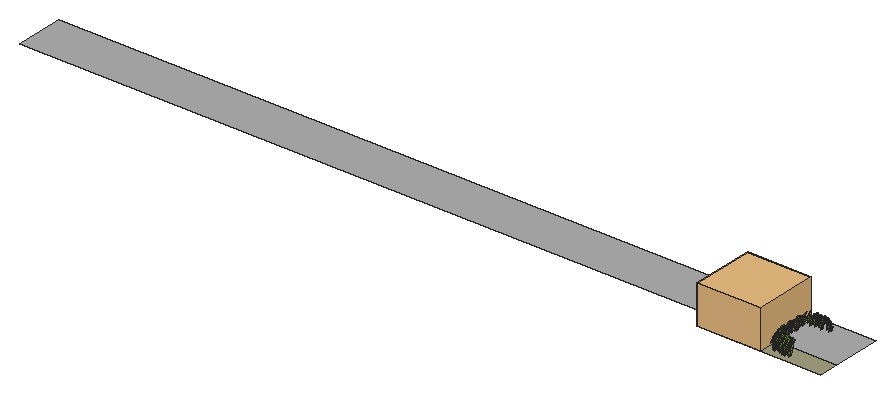
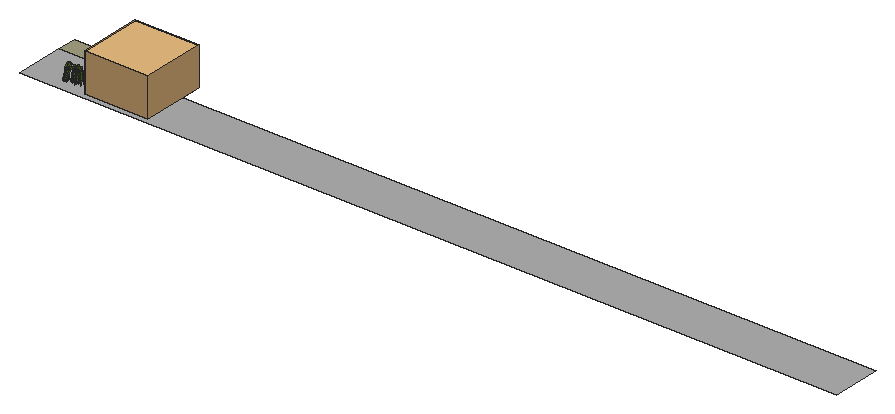
# SketchUp Ruby script. Lengths in inches.
U = 1.inch
M = Sketchup.active_model
def pt(a) = Geom::Point3d.new(a.map { |v| v * U })
def face(e, loops, mat)
  f = e.add_face(loops[0].map { |a| pt(a) })
  loops[1..].each { |l| e.add_face(l.map { |a| pt(a) }).erase! }
  f.material = f.back_material = mat if mat
  f
end
# faces: each face lists its corners as indices into pts; further lists are holes
def faces(e, pts, list, mat = nil) = list.each { |f| face(e, (f[0].is_a?(Array) ? f : [f]).map { |l| l.map { |i| pts[i] } }, mat) }
# xy, xz, yz: faces in a plane at the given z, y or x. An outline is a flat list of corners, or four numbers for a rectangle; further outlines are holes
def ring(l) = l.size == 4 ? [[l[0], l[1]], [l[2], l[1]], [l[2], l[3]], [l[0], l[3]]] : l.each_slice(2).to_a
def flat(e, list, mat, &to3) = list.each { |f| face(e, (f[0].is_a?(Array) ? f : [f]).map { |l| ring(l).map { |u, v| to3.(u, v) } }, mat) }
def xy(e, z, list, mat = nil) = flat(e, list, mat) { |x, y| [x, y, z] }
def xz(e, y, list, mat = nil) = flat(e, list, mat) { |x, z| [x, y, z] }
def yz(e, x, list, mat = nil) = flat(e, list, mat) { |y, z| [x, y, z] }
def lines(e, pts, list) = list.each { |a, b| e.add_line(pt(pts[a]), pt(pts[b])) }
# prism: a flat outline (further loops are holes) pulled along v
def prism(e, loops, v, mat = nil)
  f = face(e, loops, mat); d = Geom::Vector3d.new(v.map { |x| x * U })
  f.pushpull(f.normal.samedirection?(d) ? d.length : -d.length)
end
def box(e, o, s, mat = nil) = prism(e, [[o, [o[0] + s[0], o[1], o[2]], [o[0] + s[0], o[1] + s[1], o[2]], [o[0], o[1] + s[1], o[2]]]], [0, 0, s[2]], mat)
def at(x, y, z, deg = 0) = Geom::Transformation.translation(pt([x, y, z])) * Geom::Transformation.rotation(ORIGIN, Z_AXIS, deg.degrees)
def axes(o, x, y, z) = Geom::Transformation.new([*x, 0, *y, 0, *z, 0, *pt(o).to_a, 1])
def part(name) = M.definitions.add(name)
# library, detail: a bought-in or finely detailed component or shape, given as its bounding box
def library(name, o, s) = part(name).tap { |d| box(d.entities, o, s) }
def detail(e, o, s) = box(e.add_group.entities, o, s)
def put(e, d, t, mat = nil) = e.add_instance(d, t).tap { |i| i.material = mat if mat }
def group(e, t, mat = nil) = e.add_group.tap { |g| g.transformation = t; g.material = mat if mat }.entities
root = M.entities
M.materials.add("[0061_OliveDrab]").color = [107, 142, 35]
M.materials.add("[Carrera Marble]").color = [175, 175, 175]
M.materials.add("[Stone Coursed Rough]").color = [165, 160, 130]
c1 = library("Ornamental grass",[0,0,0],[38.24,37.94,23.16])
xy(root,543.57,[[507.27,12.12,581.95,12.12,582,41.21,90,42,89.95,12.79]],"[Carrera Marble]")
xy(root,543.57,[[581.93,0,581.95,12,581.95,12.12,507.27,12.12,507.25,0.12]],"[Stone Coursed Rough]")
p = [[554.875,33.375,546.1875],[555.06,33.4,546.1875],[554.94,33.55,543.57],[559.39,33.72,546.375],[559.6,33.65,546.375],[559.56,33.87,543.76],
  [548.13,13.96,546.65],[548.03,14.16,546.65],[547.88,13.96,544.03],[554.52,3.95,546.7],[554.3,3.97,546.7],[554.38,3.71,544.08],
  [552.98,4.9,546.76],[552.83,5.02,546.76],[552.8125,4.84,544.14],[547.99,17.08,546.71],[548,17.28,546.71],[547.83,17.1875,544.09],
  [547.81,25.01,546.74],[547.76,25.22,546.74],[547.56,25.05,544.125],[551.43,33.03,546.84],[551.61,33.14,546.84],[551.34,33.36,544.23],
  [558.59,34.56,546.78],[558.8125,34.54,546.78],[558.74,34.99,544.19],[547.64,10.6875,546.94],[547.66,10.89,546.94],[547.33,10.82,544.34],
  [555.98,33.58,546.87],[556.18,33.64,546.87],[556.02,33.8,544.26],[559.47,34.28,546.91],[559.65,34.36,546.91],[559.375,34.74,544.33],
  [560.17,34.34,546.875],[560.34,34.28,546.875],[560.42,34.74,544.29],[558.55,2.88,546.9375],[558.37,2.88,546.9375],[558.46,2.25,544.39],
  [548.33,7,546.97],[548.21,7.16,546.97],[547.78,6.72,544.42],[547.35,24.36,546.96],[547.3125,24.5625,546.96],[547.01,24.4,544.35],
  [549.7,32.17,547.01],[549.83,32.29,547.01],[549.45,32.56,544.43],[556.84,3.7,547.19],[556.625,3.77,547.19],[556.625,3.39,544.59],
  [547.6875,12.91,547.21],[547.71,13.11,547.21],[547.47,13.04,544.6],[553.87,33.84,547.23],[554.09,33.87,547.23],[553.94,34.17,544.62],
  [547.98,25.15,547.28],[548.03,25.34,547.28],[547.84,25.28,544.66],[553.67,33.4375,547.29],[553.875,33.53,547.29],[553.67,33.71,544.68],
  [551.34,4.06,547.3],[551.18,4.2,547.3],[550.85,3.65,544.75],[547.21,12.875,547.33],[547.1,13.05,547.33],[546.66,12.67,544.77],
  [547.81,15.4,547.43],[547.82,15.6,547.43],[547.6,15.51,544.8125],[546.54,15.71,547.29],[546.59,15.89,547.29],[545.85,15.98,544.77],
  [547.69,19.24,547.4],[547.66,19.4375,547.4],[547.39,19.29,544.8],[546.58,22.72,547.41],[546.5625,22.91,547.41],[546.02,22.77,544.85],
  [549.64,31.94,547.39],[549.78,32.07,547.39],[549.41,32.33,544.8],[552.55,33.67,547.42],[552.73,33.81,547.42],[552.35,34.12,544.84],
  [557.29,2.375,547.39],[557.1,2.41,547.39],[557.03,1.54,544.91],[555.79,3.96,547.51],[555.58,4.04,547.51],[555.6,3.76,544.9],
  [546.99,11.17,547.49],[547.01,11.375,547.49],[546.49,11.33,544.92],[547.1,21.32,547.48],[547.125,21.51,547.48],[546.73,21.46,544.88],
  [547.73,29.28,547.47],[547.84,29.45,547.47],[547.41,29.61,544.88],[558.51,33.59,547.5625],[558.73,33.58,547.5625],[558.625,33.77,544.94],
  [558.98,3.64,547.66],[558.77,3.67,547.66],[558.84,3.38,545.05],[546.62,20.42,547.55],[546.58,20.64,547.55],[545.91,20.39,545.02],
  [550.37,32.24,547.62],[550.54,32.34,547.62],[550.3,32.5625,545.01],[552.85,34.23,547.56],[553.0625,34.28,547.56],[552.84,34.76,544.98],
  [558.88,34.69,547.61],[559.09,34.74,547.61],[558.87,35.16,545.03],[560.95,2.5625,547.61],[560.77,2.53,547.61],[560.97,1.85,545.08],
  [546.58,25.53,547.66],[546.6,25.74,547.66],[545.95,25.67,545.11],[555.14,4.24,547.79],[554.93,4.31,547.79],[554.98,4.1,545.17],
  [552.38,4.51,547.85],[552.1875,4.59,547.85],[552.1875,4.3125,545.24],[547.5625,11.58,547.79],[547.49,11.75,547.79],[547.16,11.51,545.2],
  [547.32,12.1875,547.78],[547.375,12.38,547.78],[546.92,12.42,545.2],[546.48,14.16,547.72],[546.48,14.36,547.72],[545.76,14.26,545.2],
  [547.77,20.79,547.79],[547.75,21.01,547.79],[547.51,20.89,545.18],[547.89,24.82,547.83],[547.82,25.02,547.83],[547.65,24.85,545.21],
  [552.85,33.28,547.77],[553.04,33.38,547.77],[552.84,33.53,545.16],[561,33.55,547.86],[561.21,33.5,547.86],[561.14,33.67,545.24],
  [558.03,2.67,547.8125],[557.8125,2.62,547.8125],[558.07,1.98,545.28],[552.3,4.71,547.87],[552.09,4.75,547.87],[552.15,4.46,545.26],
  [548.19,7.04,547.88],[548.07,7.21,547.88],[547.72,6.83,545.31],[547.51,25.92,547.94],[547.46,26.125,547.94],[547.16,25.93,545.34],
  [560.18,35.33,547.83],[560.38,35.32,547.83],[560.34,36.14,545.34],[557.6875,3.67,548.05],[557.49,3.71,548.05],[557.52,3.37,545.45],
  [548.57,8.09,548.03],[548.42,8.25,548.03],[548.26,7.95,545.42],[548.13,16.84,548.05],[548.1,17.07,548.05],[547.94,16.92,545.43],
  [546.64,28.21,547.88],[546.71,28.41,547.88],[545.96,28.57,545.375],[560.52,3.79,548.12],[560.32,3.78,548.12],[560.44,3.53,545.51],
  [556.02,3.8,548.11],[555.82,3.88,548.11],[555.8,3.55,545.51],[547.55,15.5,548.14],[547.53,15.6875,548.14],[547.26,15.5625,545.54],
  [546.82,22.12,548.03],[546.86,22.31,548.03],[546.36,22.32,545.45],[549.46,32.1,548.07],[549.6,32.21,548.07],[549.17,32.63,545.52],
  [561.73,3.14,548.15],[561.51,3.09,548.15],[561.73,2.64,545.58],[548.04,14,548.17],[547.96,14.18,548.17],[547.82,14.01,545.55],
  [547.98,27.52,548.17],[547.98,27.73,548.17],[547.75,27.63,545.56],[547.37,6.89,548.12],[547.27,7.0625,548.12],[546.45,6.45,545.7],
  [547.9,26.79,548.3],[548.01,26.95,548.3],[547.73,27.03,545.69],[559.3125,35.01,548.18],[559.52,34.95,548.18],[559.59,35.68,545.66],
  [546.42,9.09,548.23],[546.38,9.3,548.23],[545.5625,9.03,545.75],[546.4,23.11,548.3],[546.4,23.33,548.3],[545.73,23.2,545.76],
  [547.9375,32.03,548.18],[548.04,32.21,548.18],[547.05,32.65,545.79],[552.25,33.93,548.41],[552.4375,33.98,548.41],[552.2,34.47,545.84],
  [558.33,35.84,548.2],[558.53,35.89,548.2],[558.21,36.91,545.81],[553.34,2.23,548.25],[553.14,2.26,548.25],[553.09,1.16,545.86],
  [560.92,2.53,548.47],[560.71,2.56,548.47],[560.73,1.89,545.93],[558.86,3.11,548.46],[558.67,3.16,548.46],[558.63,2.68,545.88],
  [557.57,2.04,548.47],[557.37,2.02,548.47],[557.54,1.23,545.98],[551.75,3.56,548.45],[551.54,3.62,548.45],[551.41,2.78,545.96],
  [557.97,3.76,548.6],[557.77,3.8,548.6],[557.83,3.52,545.98],[560.29,3.72,548.61],[560.1,3.73,548.61],[560.1875,3.48,546],
  [548.51,7.28,548.57],[548.39,7.47,548.57],[548.07,7.125,545.98],[548.29,14.96,548.61],[548.2,15.125,548.61],[548.11,14.96,545.99],
  [546.84,26.42,548.56],[546.86,26.64,548.56],[546.39,26.58,545.97],[555.38,35.11,548.5625],[555.58,35.1875,548.5625],[555.21,35.84,546.05],
  [552.23,2.64,548.52],[552.0625,2.76,548.52],[551.5,1.79,546.15],[546.44,20.76,548.62],[546.41,20.96,548.62],[545.69,20.75,546.1],
  [546.01,24.9,548.47],[546.08,25.08,548.47],[545.06,25.39,546.07],[546.71,28.26,548.58],[546.84,28.43,548.58],[546.15,28.8,546.08],
  [554.12,33.71,548.7],[554.32,33.74,548.7],[554.18,34,546.09],[554.4,34.7,548.67],[554.59,34.79,548.67],[554.19,35.39,546.14],
  [555.86,34.77,548.63],[556.04,34.82,548.63],[555.82,35.37,546.07],[553.5625,3.16,548.75],[553.375,3.25,548.75],[553.23,2.73,546.18],
  [546.57,9.7,548.76],[546.54,9.92,548.76],[545.8125,9.7,546.25],[545.53,16.1875,548.58],[545.51,16.41,548.58],[544.375,16.2,546.22],
  [554.91,32.92,548.77],[555.16,32.96,548.77],[557.51,35.57,548.64],[557.72,35.53,548.64],[557.8125,36.48,546.19],[558.86,2.49,548.84],
  [558.67,2.49,548.84],[558.76,1.86,546.29],[545.7,13.56,548.73],[545.67,13.75,548.73],[544.65,13.5,546.32],[548.14,16.22,548.89],
  [548.1,16.4,548.89],[547.97,16.28,546.27],[545.96,17.15,548.75],[546.05,17.32,548.75],[545.09,17.71,546.33],[545.81,26.47,548.68],
  [545.86,26.66,548.68],[544.82,26.87,546.28],[559.28,34.63,548.87],[559.48,34.61,548.87],[559.41,35.04,546.28],[557.74,4.12,549.07],
  [557.54,4.1,549.07],[557.65,3.94,546.45],[549.49,6.07,548.95],[549.37,6.22,548.95],[549.13,5.9,546.36],[547.83,8.52,548.97],
  [547.74,8.72,548.97],[547.37,8.43,546.39],[546.65,12.35,548.92],[546.66,12.55,548.92],[546.03,12.5,546.37],[547.63,16.52,549.06],
  [547.65,16.73,549.06],[547.35,16.65,546.45],[546.47,19.875,548.91],[546.48,20.08,548.91],[545.82,20.04,546.37],[548.03,23,548.98],
  [548.05,23.22,548.98],[547.87,23.13,546.36],[548.53,29.26,548.99],[548.61,29.43,548.99],[548.38,29.43,546.375],[559.19,33.24,548.95],
  [559.47,33.14,548.95],[556.66,2.73,548.94],[556.49,2.84,548.94],[556.09,2.03,546.48],[554.32,2.93,549.02],[554.14,2.92,549.02],
  [554.27,2.14,546.51],[556.64,3.46,549.06],[556.46,3.47,549.06],[556.54,3.14,546.46],[547.55,7.03,549],[547.48,7.21,549],
  [546.74,6.8,546.51],[546.85,19.95,549.11],[546.86,20.16,549.11],[546.3,20.06,546.55],[546.56,24.17,549.06],[546.6,24.36,549.06],
  [545.95,24.41,546.52],[549.49,30.8,549.16],[549.59,31,549.16],[549.3125,31.01,546.55],[546.47,10.28,549.03],[546.38,10.48,549.03],
  [545.55,9.98,546.58],[547.42,11.4,549.15],[547.37,11.58,549.15],[547.03,11.38,546.56],[548.66,14.15,549.21],[548.53,14.44,549.21],
  [546.8,22.22,549.15],[546.76,22.44,549.15],[546.16,22.21,546.6],[546.88,23.06,549.18],[546.82,23.27,549.18],[546.29,23.02,546.62],
  [554.63,4.58,549.24],[554.32,4.61,549.24],[549.16,7.61,549.28],[549.05,7.77,549.28],[548.93,7.5625,546.66],[548.22,9.125,549.32],
  [548.12,9.28,549.32],[547.93,9.04,546.71],[548.47,17.01,549.29],[548.48,17.3,549.29],[548.41,25.11,549.29],[548.33,25.41,549.29],
  [553.29,5.22,549.34],[553.08,5.4,549.34],[551.82,32.36,549.35],[552.07,32.52,549.35],[558.47,33.65,549.24],[558.77,33.62,549.24],
  [558.59,4.02,549.3],[558.33,4.02,549.3],[548.39,10.57,549.46],[548.42,10.86,549.46],[556.09,33.06,549.44],[556.37,33.14,549.44],
  [559.8,33.41,549.37],[560.05,33.52,549.37],[559.8125,33.5,549.34],[560.06,33.41,549.34],[549.26,7.625,549.35],[549.09,7.86,549.35],
  [548.125,24.46,549.46],[548.07,24.75,549.46],[550.34,31.46,549.46],[550.52,31.64,549.46],[557.12,4.42,549.7],[556.8125,4.52,549.7],
  [548.29,12.79,549.77],[548.32,13.09,549.77],[553.9,33.11,549.75],[554.22,33.15,549.75],[552.13,4.9,549.66],[551.9,5.1,549.66],
  [548.1875,13.4,549.71],[548.04,13.65,549.71],[547.78,15.36,549.58],[547.85,15.61,549.58],[548.46,25,549.86],[548.52,25.27,549.86],
  [553.88,32.87,549.85],[554.16,32.99,549.85],[557.6,3.78,549.58],[557.33,3.83,549.58],[548.37,15.33,549.99],[548.38,15.62,549.99],
  [548.37,19.32,549.94],[548.32,19.59,549.94],[547.72,22.78,549.78],[547.69,23.05,549.78],[550.22,31.25,549.85],[550.42,31.43,549.85],
  [553.1,32.89,549.86],[553.35,33.08,549.86],[556.05,4.53,550.06],[555.76,4.64,550.06],[548.03,11.02,549.9],[548.06,11.31,549.9],
  [547.97,21.1875,549.95],[548,21.45,549.95],[548.51,28.71,549.91],[548.67,28.96,549.91],[560.79,3.85,549.89],[560.52,3.8,549.89],
  [547.85,20.61,549.86],[547.79,20.92,549.86],[550.6875,31.57,550.13],[550.93,31.7,550.13],[558.43,33.1,550.14],[558.74,33.08,550.14],
  [558.74,33.17,549.72],[553.04,33.23,549.98],[553.34,33.3,549.98],[559.09,33.72,550.04],[559.38,33.8,550.04],[559.11,4.32,550.1875],
  [558.81,4.35,550.1875],[547.76,14.12,550.02],[547.76,14.39,550.02],[547.77,25.41,550],[547.79,25.71,550],[557.8,3.91,550.11],
  [557.49,3.84,550.11],[555.33,4.7,550.36],[555.04,4.8,550.36],[548.34,11.86,550.28],[548.24,12.11,550.28],[548.18,11.88,550.24],
  [548.26,12.16,550.24],[548.38,20.78,550.34],[548.37,21.08,550.34],[548.46,24.98,550.38],[548.36,25.26,550.38],[553.09,32.73,550.33],
  [553.36,32.88,550.33],[560.03,33.97,550.07],[560.32,33.94,550.07],[552.67,5.09,550.39],[552.39,5.2,550.39],[552.46,5.37,550.41],
  [552.17,5.42,550.41],[549.08,7.63,550.28],[548.91,7.87,550.28],[548.3,26.09,550.44],[548.22,26.38,550.44],[547.92,27.71,550.125],
  [548.02,27.99,550.125],[560.87,33.12,550.45],[561.16,33.06,550.45],[549.14,8.54,550.55],[548.9375,8.77,550.55],[547.83,21.85,550.44],
  [547.89,22.12,550.44],[557.89,4.38,550.57],[557.61,4.44,550.57],[556.34,4.45,550.64],[556.0625,4.57,550.64],[560.51,4.44,550.66],
  [560.22,4.41,550.66],[548.76,7.6875,550.2],[548.61,7.93,550.2],[548.25,15.54,550.68],[548.22,15.8,550.68],[548.61,16.88,550.63],
  [548.56,17.19,550.63],[550.08,31.21,550.46],[550.29,31.37,550.46],[553.62,3.92,550.23],[553.32,3.96,550.23],[561.55,4.13,550.58],
  [561.24,4.0625,550.58],[547.91,9.34,550.38],[547.86,9.63,550.38],[548.56,14.2,550.74],[548.44,14.45,550.74],[548.59,27.44,550.73],
  [548.6,27.75,550.73],[549.39,31.15,550.18],[549.54,31.42,550.18],[558.97,33.81,550.5],[559.26,33.74,550.5],[558.64,34.17,550.2],
  [558.92,34.23,550.2],[547.67,23.1,550.6],[547.66,23.41,550.6],[548.44,26.37,550.83],[548.6,26.59,550.83],[552.1875,4.87,550.68],
  [551.88,4.96,550.68],[552.49,32.92,550.82],[552.75,32.99,550.82],[557.47,3.54,550.625],[557.2,3.52,550.625],[561.13,3.77,550.77],
  [560.84,3.81,550.77],[553.3,4.0625,550.45],[553.0625,4.23,550.45],[559.17,4.06,550.89],[558.9,4.13,550.89],[547.5625,24.22,550.47],
  [547.66,24.47,550.47],[560.36,4.36,551.16],[560.08,4.375,551.16],[558.12,4.4,551.14],[557.84,4.45,551.14],[549.32,7.75,551.02],
  [549.15,8.01,551.02],[548.72,15.15,551.1875],[548.59,15.38,551.1875],[547.35,16.31,550.47],[547.32,16.62,550.47],[547.75,20.92,550.89],
  [547.71,21.19,550.89],[547.84,26.27,550.98],[547.87,26.58,550.98],[547.85,27.36,550.77],[548.03,27.61,550.77],[556.06,33.69,551.01],
  [556.32,33.75,551.01],[555.84,33.84,550.82],[556.11,33.95,550.82],[557.15,34.08,550.77],[557.4375,34.02,550.77],[554.1,4.14,551.125],
  [553.83,4.27,551.125],[547.4,13.77,550.72],[547.37,14.04,550.72],[547.51,16.31,550.69],[547.63,16.55,550.69],[547.44,25.9375,550.66],
  [547.52,26.2,550.66],[554.18,33.07,551.25],[554.45,33.11,551.25],[554.89,33.57,550.99],[555.16,33.69,550.99],[558.91,3.74,551.15],
  [558.65,3.74,551.15],[547.92,9.87,551.01],[547.88,10.18,551.01],[555.06,31.71,551.1],[555.37,31.76,551.1],[557.49,3.97,551.1],
  [557.26,4.12,551.1],[547.81,12.23,551.27],[547.83,12.5,551.27],[548.59,16.28,551.47],[548.53,16.54,551.47],[547.69,19.72,551.22],
  [547.72,20,551.22],[558.7,31.89,551.15],[559.05,31.77,551.15],[559.16,33.72,551.32],[559.4375,33.7,551.32],[554.29,4.24,551.29],
  [554.03,4.23,551.29],[550.17,6.58,551.4375],[550,6.8,551.4375],[548.91,7.54,551.18],[548.8125,7.79,551.18],[548.6875,8.87,551.43],
  [548.5625,9.15,551.43],[547.875,10.87,551.17],[547.75,11.15,551.17],[548.51,22.9,551.56],[548.54,23.2,551.56],[549.03,28.98,551.55],
  [549.14,29.22,551.55],[556.7,4.23,551.57],[556.4375,4.24,551.57],[557.75,4.62,551.64],[557.46,4.6,551.64],[548.3,16.43,551.59],
  [548.33,16.73,551.59],[547.92,19.89,551.51],[547.92,20.19,551.51],[547.95,22.39,551.51],[547.89,22.71,551.51],[547.74,23.85,551.38],
  [547.8,24.12,551.38],[554.82,6.15,551.34],[554.44,6.1875,551.34],[548.23,11.59,551.64],[548.15,11.85,551.64],[549.92,14.7,551.45],
  [549.75,15.05,551.45],[547.96,23.29,551.5625],[547.88,23.59,551.5625],[550.04,30.48,551.71],[550.18,30.77,551.71],[558.27,31.85,551.14],
  [558.65,31.8125,551.14],[558.61,5.96,551.07],[558.29,5.96,551.07],[554.11,6.19,551.64],[553.85,6.4,551.64],[550.84,8.75,551.12],
  [550.63,9.03,551.12],[549.66,7.89,551.84],[549.5,8.125,551.84],[548.82,9.48,551.85],[548.68,9.7,551.85],[549.83,16.91,551.53],
  [549.85,17.26,551.53],[549.88,25.45,551.4375],[549.79,25.8125,551.4375],[552.72,30.9,551.34],[553.03,31.1,551.34],[559.17,31.89,551.31],
  [559.48,31.77,551.31],[556.45,31.78,551.71],[556.79,31.88,551.71],[560.48,31.76,551.29],[560.79,31.9,551.29],[550.07,10.36,551.46],
  [550.11,10.72,551.46],[549.87,24.76,551.4],[549.8,25.12,551.4],[551.61,30.12,551.33],[551.84,30.34,551.33],[558.04,5.93,551.03],
  [557.7,5.99,551.03],[549.8,14.8125,551.17],[549.88,15.13,551.17],[557.62,5.9,551.8125],[557.25,6.02,551.8125],[553.45,6.37,551.38],
  [553.17,6.62,551.38],[549.93,14.39,551.41],[549.75,14.69,551.41],[549.82,12.59,551.89],[549.86,12.94,551.89],[549.85,22.94,551.3],
  [549.82,23.26,551.3],[551.38,29.9375,551.8],[551.62,30.16,551.8],[554.43,31.54,552.04],[554.78,31.69,552.04],[554.05,31.52,551.83],
  [554.4375,31.57,551.83],[560.48,5.99,551.38],[560.15,5.93,551.38],[549.99,10.78,551.63],[550.02,11.13,551.63],[549.87,19.55,552.08],
  [549.81,19.88,552.08],[549.875,20.97,551.49],[549.8,21.35,551.49],[549.8,24.65,552.09],[549.875,24.98,552.09],[550.09,27.62,551.6875],
  [550.29,27.92,551.6875],[554.17,31.44,551.77],[554.47,31.68,551.77],[549.84,14.09,551.62],[549.84,14.42,551.62],[549.83,15.23,552.17],
  [549.85,15.58,552.17],[549.82,20.96,551.8],[549.85,21.28,551.8],[549.83,25.26,551.625],[549.85,25.62,551.625],[553.43,31.375,551.79],
  [553.81,31.46,551.79],[559.57,31.78,551.75],[559.92,31.875,551.75],[557.36,6,551.64],[556.98,5.92,551.64],[556.6,5.89,552.23],
  [556.24,6.03,552.23],[550,26.92,551.52],[550.12,27.26,551.52],[551.47,30.08,552.15],[551.76,30.24,552.15],[558.33,31.84,552.44],
  [558.71,31.82,552.44],[559.84,31.84,551.6],[560.19,31.82,551.6],[553.97,6.3125,551.27],[553.62,6.36,551.27],[559.35,5.9375,552.24],
  [558.97,5.98,552.24],[550.75,8.86,551.46],[550.57,9.15,551.46],[549.84,11.34,552.19],[549.95,11.68,552.19],[551.45,29.95,551.27],
  [551.64,30.27,551.27],[559.12,31.79,551.21],[559.46,31.86,551.21],[550.79,8.82,551.88],[550.57,9.12,551.88],[549.9,12.48,552.3],
  [549.77,12.8,552.3],[549.85,20.8125,552.52],[549.83,21.1875,552.52],[553.76,31.39,552.48],[554.1,31.57,552.48],[555.76,5.92,552.65],
  [555.41,6.04,552.65],[553.3,6.55,552.48],[552.96,6.6875,552.48],[552.78,6.93,552.49],[552.43,7,552.49],[550.24,9.76,551.51],
  [550.17,10.12,551.51],[549.8,21.38,552.11],[549.875,21.7,552.11],[549.9,25.47,552.52],[549.78,25.8,552.52],[550.03,26.52,552.36],
  [549.93,26.88,552.36],[560.57,31.87,552.73],[560.93,31.79,552.73],[554.77,6.07,551.29],[554.48,6.27,551.29],[550.375,9.6,552.61],
  [550.12,9.88,552.61],[549.85,16.5,551.23],[549.82,16.89,551.23],[549.77,23.28,551.53],[549.9,23.59,551.53],[551.2,29.6875,552.28],
  [551.45,29.875,552.28],[558.45,31.87,552.19],[558.8,31.78,552.19],[557.28,5.97,551.6],[556.95,5.94,551.6],[561.17,6,552.38],
  [560.78,5.92,552.38],[556.98,5.89,552.73],[556.64,6.03,552.73],[558.25,5.92,552.67],[557.91,6,552.67],[549.87,17.07,552.93],
  [549.8,17.45,552.93],[549.84,23.125,552.07],[549.83,23.5,552.07],[560.39,5.98,552.79],[560.04,5.94,552.79],[552.82,6.9,552.23],
  [552.44,7.01,552.23],[549.86,14.09,551.58],[549.8125,14.43,551.58],[549.91,14.79,552.91],[549.77,15.1,552.91],[549.76,15.11,551.31],
  [549.91,15.4,551.31],[549.85,15.6875,552.74],[549.82,16.01,552.74],[549.79,25.2,551.58],[549.89,25.53,551.58],[550.14,27.34,552.84],
  [550.15,27.72,552.84],[561.46,5.94,552.22],[561.1,5.98,552.22],[549.74,25.43,552.91],[549.93,25.7,552.91],[549.75,25.93,551.89],
  [549.97,26.23,551.89],[552.95,31.11,552.67],[553.27,31.2,552.67],[556.625,31.76,552.21],[556.96,31.9,552.21],[556.64,31.87,552.08],
  [557,31.79,552.08],[559.74,5.91,552.66],[559.41,6.01,552.66],[549.86,21.21,552.42],[549.8125,21.55,552.42],[550.86,8.7,552.93],
  [550.65,9.02,552.93],[550.15,10.18,552.36],[550.09,10.56,552.36],[549.86,26.03,552.63],[549.9,26.4,552.63],[555.71,31.75,552.7],
  [556.03,31.91,552.7],[556.47,31.79,552.78],[556.79,31.87,552.78],[558.73,5.87,552.43],[558.44,6.05,552.43],[555.08,6.03,552.66],
  [554.76,6.19,552.66],[558.4,5.93,553.25],[558.05,5.99,553.25],[558.96,5.96,552.55],[558.64,5.96,552.55],[560.45,5.95,553.24],
  [560.11,5.97,553.24],[551.04,8.375,552.48],[550.92,8.68,552.48],[549.91,11.76,552.56],[549.76,12.1,552.56],[549.92,15.76,553.44],
  [549.76,16.05,553.44],[549.82,19.48,552.75],[549.85,19.83,552.75],[554.37,31.58,553.4],[554.71,31.625,553.4],[554.21,6.29,552.93],
  [553.89,6.28,552.93],[549.82,12.04,552.94],[549.85,12.38,552.94],[558.96,31.84,553.15],[559.31,31.8125,553.15],[551.5625,7.68,553.37],
  [551.34,7.95,553.37],[550.32,9.58,553.36],[550.17,9.92,553.36],[549.8,23.34,552.93],[549.875,23.66,552.93],[549.87,16.52,553.75],
  [549.8,16.84,553.75],[549.83,19.83,553.3],[549.84,20.2,553.3],[549.875,22.73,553.26],[549.8,23.11,553.26],[556.78,5.96,553.55],
  [556.45,5.96,553.55],[557.6875,5.97,553.89],[557.33,5.95,553.89],[549.88,12.04,553.63],[549.79,12.35,553.63],[549.82,16.28,553.73],
  [549.85,16.65,553.73],[549.8125,22.7,553.82],[549.86,23.07,553.82],[549.89,23.75,553.29],[549.79,24.125,553.29],[550.375,28.3125,553.71],
  [550.51,28.61,553.71],[551.37,29.79,553.86],[551.54,30.15,553.86],[550.87,8.69,554.02],[550.67,8.98,554.02],[550.1875,10.36,553.91],
  [550.01,10.62,553.91]]
faces(root,p,[[0,1,2],[3,4,5],[6,7,8],[9,10,11],[12,13,14],[15,16,17],[18,19,20],[21,22,23],
  [24,25,26],[27,28,29],[30,31,32],[33,34,35],[36,37,38],[39,40,41],[42,43,44],[45,46,47],
  [48,49,50],[51,52,53],[54,55,56],[57,58,59],[60,61,62],[63,64,65],[66,67,68],[69,70,71],
  [72,73,74],[75,76,77],[78,79,80],[81,82,83],[84,85,86],[87,88,89],[90,91,92],[93,94,95],
  [96,97,98],[99,100,101],[102,103,104],[105,106,107],[108,109,110],[111,112,113],[114,115,116],[117,118,119],
  [120,121,122],[123,124,125],[126,127,128],[129,130,131],[132,133,134],[135,136,137],[138,139,140],[141,142,143],
  [144,145,146],[147,148,149],[150,151,152],[153,154,155],[156,157,158],[159,160,161],[162,163,164],[165,166,167],
  [168,169,170],[171,172,173],[174,175,176],[177,178,179],[180,181,182],[183,184,185],[186,187,188],[189,190,191],
  [192,193,194],[195,196,197],[198,199,200],[201,202,203],[204,205,206],[207,208,209],[210,211,212],[213,214,215],
  [216,217,218],[219,220,221],[222,223,224],[225,226,227],[228,229,230],[231,232,233],[234,235,236],[237,238,239],
  [240,241,242],[243,244,245],[246,247,248],[249,250,251],[252,253,254],[255,256,257],[258,259,260],[261,262,263],
  [264,265,266],[267,268,269],[270,271,272],[273,274,275],[276,277,278],[279,280,281],[282,283,284],[285,286,287],
  [288,289,290],[291,292,293],[294,295,1,0],[296,297,298],[299,300,301],[302,303,304],[305,306,307],[308,309,310],
  [311,312,313],[314,315,316],[317,318,319],[320,321,322],[323,324,325],[326,327,328],[329,330,331],[332,333,334],
  [335,336,337],[338,339,340],[341,342,4,3],[343,344,345],[346,347,348],[349,350,351],[352,353,354],[355,356,357],
  [358,359,360],[361,362,363],[364,365,366],[367,368,369],[370,371,7,6],[372,373,374],[375,376,377],[378,379,10,9],
  [380,381,382],[383,384,385],[386,387,16,15],[388,389,19,18],[390,391,13,12],[392,393,22,21],[394,395,25,24],[396,397,40,39],
  [398,399,28,27],[400,401,31,30],[402,403,34,33],[404,405,37,36],[406,407,43,42],[408,409,46,45],[410,411,49,48],[412,413,52,51],
  [414,415,55,54],[416,417,58,57],[418,419,67,66],[420,421,70,69],[422,423,76,75],[424,425,61,60],[426,427,64,63],[428,429,91,90],
  [430,431,73,72],[432,433,79,78],[434,435,82,81],[436,437,85,84],[438,439,88,87],[440,441,94,93],[442,443,97,96],[444,445,100,99],
  [446,447,103,102],[448,449,124,123],[450,451,112,111],[452,453,115,114],[454,455,456,106,105],[457,458,118,117],[459,460,121,120],[461,462,109,108],
  [463,464,142,141],[465,466,127,126],[467,468,157,156],[469,470,130,129],[471,472,136,135],[473,474,139,138],[475,476,145,144],[477,478,148,147],
  [479,480,151,150],[481,482,169,168],[483,484,133,132],[485,486,160,159],[487,488,163,162],[489,490,166,165],[491,492,181,180],[493,494,154,153],
  [495,496,175,174],[497,498,193,192],[499,500,172,171],[501,502,187,186],[503,504,184,183],[505,506,208,207],[507,508,190,189],[509,510,178,177],
  [511,512,196,195],[513,514,232,231],[515,516,199,198],[517,518,217,216],[519,520,202,201],[521,522,205,204],[523,524,223,222],[525,526,214,213],
  [527,528,229,228],[529,530,220,219],[531,532,211,210],[533,534,244,243],[535,536,226,225],[537,538,241,240],[539,540,235,234],[541,542,265,264],
  [543,544,238,237],[545,546,271,270],[547,548,250,249],[549,550,247,246],[551,552,253,252],[553,554,256,255],[555,556,292,291],[557,558,268,267],
  [559,560,259,258],[561,562,274,273],[563,564,283,282],[565,566,262,261],[567,568,297,296],[569,570,286,285],[571,572,303,302],[573,574,309,308],
  [575,576,312,311],[577,578,277,276],[579,580,280,279],[581,582,300,299],[583,584,289,288],[585,586,295,294],[587,588,344,343],[589,590,327,326],
  [591,592,306,305],[593,594,333,332],[595,596,342,341],[597,598,315,314],[599,600,347,346],[601,602,321,320],[603,604,353,352],[605,606,324,323],
  [607,608,365,364],[609,610,336,335],[611,612,339,338],[613,614,350,349],[615,616,318,317],[617,618,330,329],[619,620,356,355],[621,622,373,372],
  [623,624,359,358],[625,626,379,378],[627,628,368,367],[629,630,371,370],[631,632,376,375],[633,634,362,361],[635,636,456,395,394],[637,638,397,396],
  [639,640,391,390],[641,642,407,406],[643,644,381,380],[645,646,384,383],[647,648,387,386],[649,650,389,388],[651,652,393,392],[653,654,405,404],
  [655,656,401,400],[657,658,403,402],[659,660,399,398],[661,662,409,408],[663,664,411,410],[665,666,429,428],[667,668,423,422],[669,670,413,412],
  [671,672,419,418],[673,674,421,420],[675,676,415,414],[677,678,435,434],[679,680,437,436],[681,682,427,426],[683,684,417,416],[685,686,449,448],
  [687,688,443,442],[689,690,433,432],[691,692,451,450],[693,694,425,424],[695,696,447,446],[697,698,439,438],[699,700,464,463],[701,702,431,430],
  [703,704,445,444],[705,706,466,465],[707,708,458,457],[709,710,460,459],[711,712,468,467],[713,714,441,440],[715,716,492,491],[717,718,453,452],
  [719,720,455,454],[721,722,482,481],[723,724,514,513],[725,726,462,461],[727,728,506,505],[729,730,474,473],[731,732,524,523],[733,734,528,527],
  [735,736,488,487],[737,738,472,471],[739,740,476,475],[741,742,480,479],[743,744,470,469],[745,746,484,483],[747,748,486,485],[749,750,518,517],
  [751,752,498,497],[753,754,478,477],[755,756,490,489],[757,758,494,493],[759,760,542,541],[761,762,496,495],[763,764,556,555],[765,766,546,545],
  [767,768,512,511],[769,770,526,525],[771,772,538,537],[773,774,516,515],[775,776,502,501],[777,778,500,499],[779,780,510,509],[781,782,530,529],
  [783,784,504,503],[785,786,534,533],[787,788,572,571],[789,790,520,519],[791,792,574,573],[793,794,508,507],[795,796,576,575],[797,798,522,521],
  [799,800,540,539],[801,802,532,531],[803,804,562,561],[805,806,536,535],[807,808,566,565],[809,810,568,567],[811,812,544,543],[813,814,558,557],
  [815,816,552,551],[817,818,584,583],[819,820,560,559],[821,822,580,579],[823,824,564,563],[825,826,588,587],[827,828,570,569],[829,830,550,549],
  [831,832,582,581],[833,834,548,547],[835,836,604,603],[837,838,608,607],[839,840,554,553],[841,842,594,593],[843,844,578,577],[845,846,600,599],
  [847,848,590,589],[849,850,598,597],[851,852,602,601],[853,854,606,605],[855,856,624,623],[857,858,592,591],[859,860,620,619],[861,862,622,621],
  [863,864,614,613],[865,866,616,615],[867,868,628,627],[869,870,618,617],[871,872,610,609],[873,874,632,631],[875,876,612,611],[877,878,634,633],
  [879,880,644,643],[881,882,646,645]],"[0061_OliveDrab]")
put(root,c1,at(507.25,0.12,543.57),"[0061_OliveDrab]")
